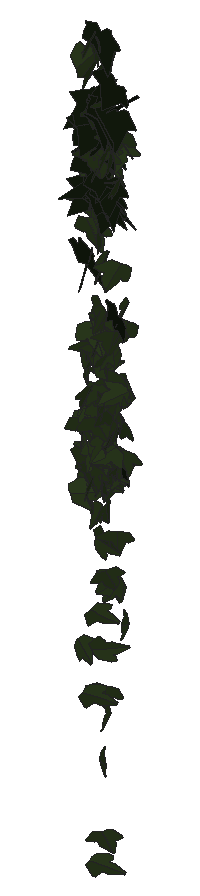
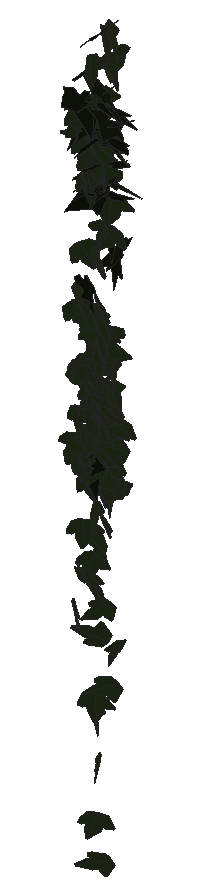
# SketchUp Ruby script. Lengths in inches.
U = 1.inch
M = Sketchup.active_model
def pt(a) = Geom::Point3d.new(a.map { |v| v * U })
def face(e, loops, mat)
  f = e.add_face(loops[0].map { |a| pt(a) })
  loops[1..].each { |l| e.add_face(l.map { |a| pt(a) }).erase! }
  f.material = f.back_material = mat if mat
  f
end
# faces: each face lists its corners as indices into pts; further lists are holes
def faces(e, pts, list, mat = nil) = list.each { |f| face(e, (f[0].is_a?(Array) ? f : [f]).map { |l| l.map { |i| pts[i] } }, mat) }
# xy, xz, yz: faces in a plane at the given z, y or x. An outline is a flat list of corners, or four numbers for a rectangle; further outlines are holes
def ring(l) = l.size == 4 ? [[l[0], l[1]], [l[2], l[1]], [l[2], l[3]], [l[0], l[3]]] : l.each_slice(2).to_a
def flat(e, list, mat, &to3) = list.each { |f| face(e, (f[0].is_a?(Array) ? f : [f]).map { |l| ring(l).map { |u, v| to3.(u, v) } }, mat) }
def xy(e, z, list, mat = nil) = flat(e, list, mat) { |x, y| [x, y, z] }
def xz(e, y, list, mat = nil) = flat(e, list, mat) { |x, z| [x, y, z] }
def yz(e, x, list, mat = nil) = flat(e, list, mat) { |y, z| [x, y, z] }
def lines(e, pts, list) = list.each { |a, b| e.add_line(pt(pts[a]), pt(pts[b])) }
# prism: a flat outline (further loops are holes) pulled along v
def prism(e, loops, v, mat = nil)
  f = face(e, loops, mat); d = Geom::Vector3d.new(v.map { |x| x * U })
  f.pushpull(f.normal.samedirection?(d) ? d.length : -d.length)
end
def box(e, o, s, mat = nil) = prism(e, [[o, [o[0] + s[0], o[1], o[2]], [o[0] + s[0], o[1] + s[1], o[2]], [o[0], o[1] + s[1], o[2]]]], [0, 0, s[2]], mat)
def at(x, y, z, deg = 0) = Geom::Transformation.translation(pt([x, y, z])) * Geom::Transformation.rotation(ORIGIN, Z_AXIS, deg.degrees)
def axes(o, x, y, z) = Geom::Transformation.new([*x, 0, *y, 0, *z, 0, *pt(o).to_a, 1])
def part(name) = M.definitions.add(name)
# library, detail: a bought-in or finely detailed component or shape, given as its bounding box
def library(name, o, s) = part(name).tap { |d| box(d.entities, o, s) }
def detail(e, o, s) = box(e.add_group.entities, o, s)
def put(e, d, t, mat = nil) = e.add_instance(d, t).tap { |i| i.material = mat if mat }
def group(e, t, mat = nil) = e.add_group.tap { |g| g.transformation = t; g.material = mat if mat }.entities
root = M.entities
M.materials.add("1026 AP 7946 SUNNY SIDE UP").color = [254, 231, 186]
M.materials.add("efeu1").color = [18, 25, 13]
M.materials.add("efeu2").color = [43, 57, 29]
c1 = part("ivyleaf_10")
p = [[0,0.5,-0.03],[-0.0625,2.02,-0.43],[-0.19,2.01,-0.46],[-0.54,1.05,-0.29],[-0.52,0.625,-0.18],[-0.83,0.76,-0.28],
  [-1.16,0.64,-0.33],[-1.15,0.33,-0.24],[-0.77,-0.39,0.02],[-0.3,-0.51,0.16],[0.04,-0.48,0.23],[-0.02,2.01,-0.4375],
  [-0.06,2.01,-0.43],[0.04,-0.49,0.23],[0.67,-0.49,0.14],[1.38,0.36,-0.2],[1.375,0.51,-0.24],[0.81,0.65,-0.19],
  [0.62,0.59,-0.15],[0.6,1.09,-0.28],[0.5,1.23,-0.31]]
faces(c1.entities,p,[[0,1,2,3,4,5,6,7,8,9,10],[11,12,0,13,14,15,16,17,18,19,20]],"efeu2")
c2 = part("ivyleaf_9")
p = [[1.54,2.16,1.25],[1.36,2.04,1.19],[-0.21,0.99,0.68],[-0.71,1.11,0.82],[-0.85,0.86,0.67],[-0.8,0.17,0.21],
  [-0.9,-0.01,0.1],[-0.67,-0.16,-0.02],[-0.08,-0.08,-0.05],[-0.03,-0.6,-0.4],[0.65,-0.88,-0.66],[0.83,-0.6,-0.49],
  [1.29,-0.42,-0.43],[1.8125,-0.07,-0.26],[1.21,0.44,0.15]]
faces(c2.entities,p,[[0,1,2,3,4,5,6,7,8,9,10,11,12,13,14]],"efeu1")
put(root,c1,axes([105.44,212.83,261.08],[-0.22128,-0.17573,0.01533],[0.00706,-0.02387,-0.2313],[0.27735,-0.1396,0.01812]),"1026 AP 7946 SUNNY SIDE UP")
put(root,c1,axes([105.27,212.93,260.67],[0.07124,-0.10081,0.19446],[0.19545,-0.14537,-0.11123],[0.27488,0.12949,0.0287]),"1026 AP 7946 SUNNY SIDE UP")
put(root,c1,axes([105.36,212.74,259.4],[-0.02708,0.1432,-0.1626],[-0.00095,-0.1592,-0.1489],[-0.33605,-0.01109,0.01352]),"1026 AP 7946 SUNNY SIDE UP")
put(root,c1,axes([105.4375,212.62,260.73],[0.03044,-0.01682,-0.23325],[-0.00065,0.22714,-0.0161],[0.35685,0.00185,0.01987]),"1026 AP 7946 SUNNY SIDE UP")
put(root,c1,axes([105.38,212.6,254.75],[0.00854,0.19841,0.07647],[-0.00793,0.07323,-0.20393],[-0.33238,0.00335,0.00683]),"1026 AP 7946 SUNNY SIDE UP")
put(root,c2,axes([105.5,212.76,266],[0.09763,0.17061,0.17604],[-0.03799,0.179,-0.17502],[-0.37671,0.02617,0.06327]),"1026 AP 7946 SUNNY SIDE UP")
put(root,c1,axes([105.26,212.79,258.43],[-0.15952,0.09823,-0.20296],[0.19847,-0.15252,-0.14578],[-0.28456,-0.16144,0.0121]),"1026 AP 7946 SUNNY SIDE UP")
put(root,c1,axes([105.46,212.78,264.3],[-0.30335,-0.14355,-0.00701],[0.02705,-0.01312,-0.24688],[0.22429,-0.19257,0.02029]),"1026 AP 7946 SUNNY SIDE UP")
put(root,c1,axes([105.53,212.83,258.88],[-0.20843,-0.10504,0.13226],[-0.05293,-0.14457,-0.15778],[0.25615,-0.11535,0.07502]),"1026 AP 7946 SUNNY SIDE UP")
put(root,c1,axes([105.48,212.68,260.21],[0.01512,-0.21436,0.03388],[0.00431,-0.03402,-0.22125],[0.34127,0.00993,0.00129]),"1026 AP 7946 SUNNY SIDE UP")
put(root,c1,axes([105.39,212.64,259.49],[-0.30371,-0.07569,-0.09097],[0.14534,0.00264,-0.21163],[0.11014,-0.21218,0.02842]),"1026 AP 7946 SUNNY SIDE UP")
put(root,c2,axes([105.56,212.89,264.43],[-0.3257,-0.11911,0.03771],[-0.02627,-0.04513,-0.24442],[0.19449,-0.20557,0.03014]),"1026 AP 7946 SUNNY SIDE UP")
put(root,c1,axes([105.47,212.86,261.24],[-0.33841,0.04416,-0.01506],[0.01648,-0.02262,-0.22553],[-0.07139,-0.21454,0.01935]),"1026 AP 7946 SUNNY SIDE UP")
put(root,c1,axes([105.55,212.65,257.8],[0.00414,0.04895,-0.20902],[-0.08657,0.19617,0.0491],[0.317,0.05293,0.01614]),"1026 AP 7946 SUNNY SIDE UP")
put(root,c2,axes([105.64,212.4,262.97],[-0.0648,0.0313,-0.2871],[-0.3536,0.16492,0.05427],[0.26394,0.22862,0.00222]),"1026 AP 7946 SUNNY SIDE UP")
put(root,c1,axes([105.51,212.99,258.33],[0.25702,0.11622,0.03653],[-0.07124,0.00431,0.20442],[0.17696,-0.16706,0.02924]),"1026 AP 7946 SUNNY SIDE UP")
put(root,c2,axes([105.625,212.85,266.29],[-0.38246,-0.04765,0.01537],[-0.01648,-0.02519,-0.25441],[0.0769,-0.2424,0.02193]),"1026 AP 7946 SUNNY SIDE UP")
put(root,c2,axes([105.28,212.68,263.21],[0.23413,-0.2247,-0.02069],[-0.02429,0.01232,-0.27755],[0.35372,0.14958,-0.00537]),"1026 AP 7946 SUNNY SIDE UP")
put(root,c1,axes([105.34,212.82,259.53],[0.32917,-0.00311,0.08997],[0.13655,-0.01825,-0.21519],[0.01555,0.2261,-0.0148]),"1026 AP 7946 SUNNY SIDE UP")
put(root,c1,axes([105.41,212.52,267.25],[0.06637,0.06134,-0.28287],[0.15017,0.25842,0.07602],[0.41669,-0.1029,0.01766]),"1026 AP 7946 SUNNY SIDE UP")
put(root,c1,axes([105.55,212.86,261.93],[0.16171,-0.18218,-0.10114],[-0.06315,0.0888,-0.21485],[0.31844,0.11013,0.00875]),"1026 AP 7946 SUNNY SIDE UP")
put(root,c1,axes([105.43,212.82,263.68],[-0.35081,0.02377,-0.08698],[0.11461,-0.07874,-0.22136],[-0.0771,-0.22522,0.06672]),"1026 AP 7946 SUNNY SIDE UP")
put(root,c1,axes([105.54,212.73,267.17],[0.10726,-0.24656,0.04116],[0.00872,-0.04137,-0.26373],[0.39302,0.06821,-0.00538]),"1026 AP 7946 SUNNY SIDE UP")
put(root,c1,axes([105.57,212.64,267.8125],[0.11867,-0.25043,-0.01937],[-0.01412,0.01544,-0.26933],[0.39448,0.07589,-0.00382]),"1026 AP 7946 SUNNY SIDE UP")
put(root,c2,axes([105.51,212.83,265.83],[-0.1649,-0.21075,0.08769],[-0.02069,-0.08926,-0.24151],[0.35749,-0.10237,0.02647]),"1026 AP 7946 SUNNY SIDE UP")
put(root,c1,axes([105.53,212.91,257.57],[0.22071,-0.14882,0.00739],[-0.00058,-0.01136,-0.21065],[0.23435,0.14013,-0.00748]),"1026 AP 7946 SUNNY SIDE UP")
put(root,c1,axes([105.55,212.68,258.3],[0.13075,-0.18767,0.04393],[0.02963,-0.03946,-0.2117],[0.30154,0.08526,0.00175]),"1026 AP 7946 SUNNY SIDE UP")
put(root,c2,axes([105.37,212.94,264.71],[0.17879,-0.21134,0.0306],[0.00684,-0.03271,-0.24713],[0.33577,0.1132,-0.01126]),"1026 AP 7946 SUNNY SIDE UP")
put(root,c1,axes([105.59,212.82,265.04],[0.1143,-0.21643,-0.10668],[-0.01175,0.10484,-0.23328],[0.37624,0.06902,0.02513]),"1026 AP 7946 SUNNY SIDE UP")
put(root,c1,axes([105.59,212.91,261.2],[0.09608,-0.21652,0.00671],[0.00368,-0.00738,-0.23181],[0.34065,0.06115,0.00061]),"1026 AP 7946 SUNNY SIDE UP")
put(root,c1,axes([105.625,213.03,253.6875],[-0.29514,-0.07377,0.01932],[-0.01723,-0.0243,-0.20703],[0.11861,-0.18711,0.01799]),"1026 AP 7946 SUNNY SIDE UP")
put(root,c1,axes([105.625,212.84,259.79],[0.10771,-0.20456,-0.06023],[-0.03818,0.05227,-0.22184],[0.33184,0.07241,-0.00597]),"1026 AP 7946 SUNNY SIDE UP")
put(root,c2,axes([105.79,212.77,266.65],[-0.18898,0.21599,0.03996],[-0.04326,0.02763,-0.25425],[-0.342,-0.12285,0.01008]),"1026 AP 7946 SUNNY SIDE UP")
put(root,c1,axes([105.6,212.85,259.82],[0.30425,-0.08417,-0.03252],[-0.05238,0.00122,-0.21702],[0.13101,0.19597,-0.01126]),"1026 AP 7946 SUNNY SIDE UP")
put(root,c2,axes([105.81,212.68,264.7],[-0.35867,0.08132,-0.01111],[-0.03158,-0.08747,-0.23251],[-0.12516,-0.21096,0.0905]),"1026 AP 7946 SUNNY SIDE UP")
put(root,c1,axes([105.54,212.78,259.67],[0.21054,0.16646,-0.02597],[-0.01059,-0.02809,-0.21988],[-0.26474,0.1335,-0.01185]),"1026 AP 7946 SUNNY SIDE UP")
put(root,c1,axes([105.38,212.49,258.05],[0.09678,-0.02241,-0.2198],[0.29038,0.11825,0.0428],[0.17129,-0.18781,0.05163]),"1026 AP 7946 SUNNY SIDE UP")
put(root,c1,axes([105.54,212.96,261.38],[0.2227,-0.16798,0.02163],[0.06951,0.00903,-0.22263],[0.25715,0.14304,0.04145]),"1026 AP 7946 SUNNY SIDE UP")
put(root,c2,axes([105.49,212.85,265.07],[-0.07743,-0.23381,-0.06941],[0.06074,0.059,-0.24448],[0.37717,-0.0575,0.02512]),"1026 AP 7946 SUNNY SIDE UP")
put(root,c2,axes([105.8,212.6875,265.68],[-0.25575,0.18251,-0.01538],[-0.0019,-0.02242,-0.25146],[-0.28807,-0.16189,0.01531]),"1026 AP 7946 SUNNY SIDE UP")
put(root,c1,axes([105.69,212.92,259.87],[0.08485,-0.16349,-0.13708],[-0.07215,0.12397,-0.1766],[0.32256,0.07074,-0.00344]),"1026 AP 7946 SUNNY SIDE UP")
put(root,c1,axes([105.62,212.57,258.61],[-0.32865,0.03345,-0.02605],[0.03395,-0.02551,-0.21707],[-0.05674,-0.20901,0.02105]),"1026 AP 7946 SUNNY SIDE UP")
put(root,c1,axes([105.35,212.79,258.18],[0.03251,0.02249,0.24878],[0.30742,0.14166,-0.03002],[-0.22534,0.19651,-0.00507]),"1026 AP 7946 SUNNY SIDE UP")
put(root,c1,axes([105.65,212.72,261.35],[0.13984,-0.21069,-0.07232],[-0.01219,0.07134,-0.2343],[0.34839,0.08706,0.02083]),"1026 AP 7946 SUNNY SIDE UP")
put(root,c1,axes([105.79,212.84,261.62],[-0.30331,0.05361,0.11483],[-0.19069,-0.04409,-0.19515],[-0.03598,-0.21822,0.06623]),"1026 AP 7946 SUNNY SIDE UP")
put(root,c1,axes([105.68,212.84,261.125],[-0.18243,-0.18461,0.0588],[-0.00916,-0.06441,-0.22309],[0.30419,-0.11266,0.02855]),"1026 AP 7946 SUNNY SIDE UP")
put(root,c1,axes([105.47,212.87,264.99],[0.28176,0.13939,0.10132],[0.13664,0.04683,-0.23308],[-0.22999,0.19858,-0.01435]),"1026 AP 7946 SUNNY SIDE UP")
put(root,c1,axes([105.71,212.8,252.27],[-0.09485,0.12016,0.15773],[-0.1359,0.12629,-0.13706],[-0.27326,-0.10451,0.01341]),"1026 AP 7946 SUNNY SIDE UP")
put(root,c1,axes([105.61,212.85,258.3],[-0.13688,0.17784,-0.05397],[0.01805,-0.05371,-0.20386],[-0.2914,-0.08686,0.01273]),"1026 AP 7946 SUNNY SIDE UP")
put(root,c1,axes([105.67,212.84,258.21],[0.10369,-0.20167,-0.01],[-0.00579,0.00781,-0.21854],[0.31734,0.06604,-0.00072]),"1026 AP 7946 SUNNY SIDE UP")
put(root,c1,axes([105.7,212.62,267.71],[0.23168,-0.17596,-0.13413],[-0.04584,0.13861,-0.22793],[0.34018,0.13852,0.06063]),"1026 AP 7946 SUNNY SIDE UP")
put(root,c2,axes([105.46,212.87,265.7],[-0.13789,-0.1389,-0.19304],[0.28735,0.08225,-0.15107],[0.22632,-0.18906,0.07419]),"1026 AP 7946 SUNNY SIDE UP")
put(root,c1,axes([105.7,212.84,261.43],[-0.28965,-0.12276,-0.00066],[0.01501,-0.01443,-0.22744],[0.19245,-0.18365,0.01675]),"1026 AP 7946 SUNNY SIDE UP")
put(root,c1,axes([105.65,212.69,259],[0.16619,0.16723,-0.09234],[-0.05843,-0.08348,-0.20392],[-0.29329,0.11139,-0.0117]),"1026 AP 7946 SUNNY SIDE UP")
put(root,c1,axes([105.68,212.92,259.67],[-0.28669,-0.11341,-0.01529],[0.04923,-0.02385,-0.21808],[0.17284,-0.18131,0.03676]),"1026 AP 7946 SUNNY SIDE UP")
put(root,c1,axes([105.7,212.77,259.82],[0.16729,0.16243,-0.09678],[-0.10342,-0.06998,-0.19985],[-0.2771,0.12418,0.01616]),"1026 AP 7946 SUNNY SIDE UP")
put(root,c1,axes([105.64,212.81,259.72],[0.36752,0.02151,-0.00868],[-0.01043,-0.02089,-0.24103],[-0.03487,0.23295,-0.01942]),"1026 AP 7946 SUNNY SIDE UP")
put(root,c1,axes([105.47,212.55,258.98],[-0.19521,-0.02606,-0.19883],[0.3051,0.00098,-0.1288],[0.02348,-0.22935,0.02068]),"1026 AP 7946 SUNNY SIDE UP")
put(root,c1,axes([105.54,212.73,261.52],[0.29677,0.12947,0.07025],[0.10553,0.02096,-0.23477],[-0.20385,0.19933,-0.01927]),"1026 AP 7946 SUNNY SIDE UP")
put(root,c1,axes([105.88,212.7,260.24],[-0.26732,-0.01176,0.14184],[-0.20106,-0.06964,-0.16911],[0.08266,-0.20743,0.04738]),"1026 AP 7946 SUNNY SIDE UP")
put(root,c1,axes([105.66,212.77,259.4],[0.04673,-0.20678,-0.04953],[0.0857,0.05322,-0.20583],[0.3222,0.01584,0.06193]),"1026 AP 7946 SUNNY SIDE UP")
put(root,c1,axes([105.76,212.91,265.17],[-0.22954,-0.18934,0.05011],[-0.00328,-0.06051,-0.24407],[0.30779,-0.14185,0.03477]),"1026 AP 7946 SUNNY SIDE UP")
put(root,c1,axes([105.68,212.68,263.65],[0.17551,-0.17899,-0.13159],[0.0416,0.15213,-0.19649],[0.34231,0.07328,0.09134]),"1026 AP 7946 SUNNY SIDE UP")
put(root,c1,axes([105.72,213,267.26],[0.01297,-0.24213,-0.06823],[0.03226,0.06532,-0.24818],[0.39282,0.00263,0.02263]),"1026 AP 7946 SUNNY SIDE UP")
put(root,c1,axes([105.71,212.9,257.6875],[0.03121,-0.19628,-0.06063],[0.05312,0.06036,-0.19906],[0.31729,0.0092,0.03929]),"1026 AP 7946 SUNNY SIDE UP")
put(root,c1,axes([105.76,212.67,266.39],[-0.07212,-0.25224,0.00935],[0.00499,-0.01125,-0.26413],[0.39694,-0.04569,0.00502]),"1026 AP 7946 SUNNY SIDE UP")
put(root,c1,axes([105.68,212.9,263.01],[0.18163,-0.17997,0.11615],[0.07411,-0.10461,-0.22038],[0.32648,0.12386,-0.01459]),"1026 AP 7946 SUNNY SIDE UP")
put(root,c1,axes([105.73,212.71,264.68],[0.20142,-0.2197,0.05315],[0.0154,-0.05529,-0.26159],[0.35498,0.12706,-0.01881]),"1026 AP 7946 SUNNY SIDE UP")
put(root,c2,axes([105.58,213.02,265.67],[0.10509,-0.21914,-0.08396],[-0.02049,0.07985,-0.23532],[0.36639,0.06732,0.01092]),"1026 AP 7946 SUNNY SIDE UP")
put(root,c1,axes([105.78,212.6,265.4],[-0.35455,-0.1182,-0.01023],[0.02885,-0.01514,-0.26139],[0.18419,-0.22517,0.02125]),"1026 AP 7946 SUNNY SIDE UP")
put(root,c2,axes([105.86,212.92,258.6875],[0.22062,0.00839,-0.2021],[-0.30364,-0.03807,-0.14415],[-0.0563,0.2382,-0.01449]),"1026 AP 7946 SUNNY SIDE UP")
put(root,c1,axes([105.6,212.56,253.79],[-0.11231,-0.06712,-0.1954],[0.25288,0.10123,-0.0989],[0.18916,-0.17518,0.0162]),"1026 AP 7946 SUNNY SIDE UP")
put(root,c1,axes([105.83,212.81,253.3],[0.09239,-0.18145,-0.09849],[-0.05036,0.08902,-0.19595],[0.31778,0.06686,-0.00242]),"1026 AP 7946 SUNNY SIDE UP")
put(root,c1,axes([105.84,212.67,258.41],[-0.15414,0.16749,0.06277],[-0.11099,0.02624,-0.19419],[-0.25677,-0.11189,0.04626]),"1026 AP 7946 SUNNY SIDE UP")
put(root,c1,axes([105.67,212.67,255.52],[-0.1223,-0.10744,-0.17196],[0.19701,0.11165,-0.13402],[0.24107,-0.14575,0.02228]),"1026 AP 7946 SUNNY SIDE UP")
put(root,c2,axes([105.66,212.84,267.83],[0.01478,-0.25847,0.0371],[-0.00259,-0.03757,-0.26665],[0.41066,0.00907,-0.00302]),"1026 AP 7946 SUNNY SIDE UP")
put(root,c1,axes([105.82,212.66,261.93],[0.20302,-0.18658,-0.03932],[-0.03314,0.03055,-0.23357],[0.29728,0.13082,0.00082]),"1026 AP 7946 SUNNY SIDE UP")
put(root,c1,axes([105.88,212.83,258.56],[-0.14367,0.1788,0.05168],[-0.14008,0.00572,-0.19205],[-0.25573,-0.10359,0.07617]),"1026 AP 7946 SUNNY SIDE UP")
put(root,c1,axes([105.78,212.75,261.13],[0.31645,-0.10306,0.01238],[0.00359,-0.02309,-0.2322],[0.16322,0.20032,-0.01889]),"1026 AP 7946 SUNNY SIDE UP")
put(root,c1,axes([105.55,212.92,256.89],[-0.05227,0.02222,0.24345],[0.35872,-0.06242,0.03876],[0.10231,0.23021,-0.01153]),"1026 AP 7946 SUNNY SIDE UP")
put(root,c1,axes([105.63,212.74,250.11],[-0.10531,-0.05523,-0.18963],[0.27345,0.06477,-0.08497],[0.12749,-0.18455,0.02562]),"1026 AP 7946 SUNNY SIDE UP")
put(root,c2,axes([105.6875,212.76,266.13],[0.03173,-0.23224,0.09141],[-0.00011,-0.09035,-0.24056],[0.39166,0.01879,-0.00747]),"1026 AP 7946 SUNNY SIDE UP")
put(root,c1,axes([105.87,212.55,260.13],[0.18328,-0.15919,-0.10779],[-0.04038,0.10738,-0.19886],[0.29602,0.11321,0.03962]),"1026 AP 7946 SUNNY SIDE UP")
put(root,c1,axes([105.88,212.92,258.26],[-0.14719,-0.1728,0.05221],[-0.00739,-0.05585,-0.20154],[0.28349,-0.09117,0.02186]),"1026 AP 7946 SUNNY SIDE UP")
put(root,c1,axes([105.71,212.78,258.86],[0.18207,-0.10262,0.16717],[0.17426,-0.11984,-0.15968],[0.24746,0.15989,-0.01055]),"1026 AP 7946 SUNNY SIDE UP")
put(root,c1,axes([105.96,212.87,256.18],[0.28464,-0.1046,-0.12753],[-0.17573,0.0526,-0.21488],[0.18357,0.21255,-0.00796]),"1026 AP 7946 SUNNY SIDE UP")
put(root,c1,axes([105.875,212.7,259.2],[0.14901,0.13785,-0.14507],[-0.11519,-0.12134,-0.17292],[-0.2886,0.11961,-0.00589]),"1026 AP 7946 SUNNY SIDE UP")
put(root,c1,axes([105.8,212.55,259.7],[-0.25755,-0.16208,-0.09159],[0.12527,0.04394,-0.23593],[0.26153,-0.18066,0.02282]),"1026 AP 7946 SUNNY SIDE UP")
put(root,c1,axes([105.86,212.96,258.51],[-0.07485,-0.11851,0.16217],[0.0293,-0.16458,-0.12228],[0.30929,-0.01309,0.05083]),"1026 AP 7946 SUNNY SIDE UP")
put(root,c1,axes([105.93,212.91,260.09],[0.12838,-0.16306,-0.12463],[-0.08839,0.10611,-0.18723],[0.30588,0.0991,-0.00179]),"1026 AP 7946 SUNNY SIDE UP")
put(root,c1,axes([105.9,212.84,264.65],[-0.15409,-0.22399,0.00098],[0.01203,-0.00577,-0.25172],[0.35201,-0.09785,0.00903]),"1026 AP 7946 SUNNY SIDE UP")
put(root,c1,axes([105.8125,212.65,260.82],[0.03532,-0.00074,0.23556],[0.00505,0.22974,0.00179],[-0.35952,0.00316,0.02316]),"1026 AP 7946 SUNNY SIDE UP")
put(root,c1,axes([105.89,212.93,259.28],[-0.00796,-0.20859,-0.04954],[0.01367,0.04668,-0.21454],[0.33589,-0.00684,0.00756]),"1026 AP 7946 SUNNY SIDE UP")
put(root,c1,axes([105.64,212.9375,258.56],[0.17513,0.0272,0.17597],[0.26014,0.04189,-0.11786],[-0.07853,0.19944,0.002]),"1026 AP 7946 SUNNY SIDE UP")
put(root,c1,axes([105.93,212.73,260.68],[-0.34339,-0.00294,0.02329],[-0.0349,-0.023,-0.22393],[0.00829,-0.21835,0.02198]),"1026 AP 7946 SUNNY SIDE UP")
put(root,c1,axes([105.87,212.87,260.19],[-0.08582,-0.20689,-0.03054],[0.05828,0.01936,-0.21805],[0.32317,-0.05844,0.03121]),"1026 AP 7946 SUNNY SIDE UP")
put(root,c1,axes([105.89,212.76,265.46],[0.11715,-0.22431,0.07234],[0.01978,-0.07109,-0.24369],[0.36966,0.07489,-0.00989]),"1026 AP 7946 SUNNY SIDE UP")
put(root,c1,axes([105.89,212.92,261.78],[-0.2745,0.13573,-0.02631],[0.00647,-0.03726,-0.22636],[-0.2173,-0.17257,0.02649]),"1026 AP 7946 SUNNY SIDE UP")
put(root,c1,axes([105.65,212.87,265.32],[0.28008,0.01213,0.1789],[0.27191,0.01535,-0.18382],[-0.0305,0.24824,0.00409]),"1026 AP 7946 SUNNY SIDE UP")
put(root,c2,axes([105.7,212.85,264.4],[0.36284,-0.07611,-0.0014],[-0.01432,-0.02466,-0.249],[0.11883,0.22944,-0.02573]),"1026 AP 7946 SUNNY SIDE UP")
put(root,c1,axes([105.94,212.88,260.52],[-0.14462,-0.20128,0.02611],[0.00688,-0.03104,-0.22751],[0.31915,-0.09054,0.01673]),"1026 AP 7946 SUNNY SIDE UP")
put(root,c2,axes([106.03,212.95,266.38],[-0.02246,0.24952,-0.01696],[-0.00298,-0.01802,-0.25756],[-0.39334,-0.01411,0.00292]),"1026 AP 7946 SUNNY SIDE UP")
put(root,c1,axes([106.01,212.66,259.11],[0.29327,-0.01055,-0.11936],[-0.18281,-0.01234,-0.19181],[0.00383,0.21919,-0.01525]),"1026 AP 7946 SUNNY SIDE UP")
put(root,c1,axes([105.93,213,258.64],[0.16954,-0.17442,-0.00351],[-0.00202,0.00205,-0.21123],[0.27427,0.10783,0.00062]),"1026 AP 7946 SUNNY SIDE UP")
put(root,c2,axes([105.88,212.78,264.38],[-0.11526,-0.22783,0.04637],[-0.01929,-0.04469,-0.24681],[0.36505,-0.07429,0.0016]),"1026 AP 7946 SUNNY SIDE UP")
put(root,c1,axes([105.9,212.95,258.52],[0.31181,-0.04079,0.0034],[-0.00037,-0.01859,-0.20783],[0.06437,0.19746,-0.01765]),"1026 AP 7946 SUNNY SIDE UP")
put(root,c2,axes([105.8,212.75,266.34],[0.02956,-0.25303,0.03258],[0.0012,-0.03309,-0.26158],[0.40125,0.01874,-0.00162]),"1026 AP 7946 SUNNY SIDE UP")
put(root,c1,axes([105.92,212.6,250.86],[-0.23222,-0.12732,-0.06276],[0.0878,0.02714,-0.20011],[0.2033,-0.15716,0.01474]),"1026 AP 7946 SUNNY SIDE UP")
put(root,c1,axes([106,212.86,265.72],[-0.27678,-0.17845,0.01127],[0.00776,-0.02161,-0.25763],[0.28111,-0.1751,0.0182]),"1026 AP 7946 SUNNY SIDE UP")
put(root,c2,axes([105.8125,212.58,264.59],[0.16154,-0.18341,-0.14312],[-0.06961,0.13239,-0.21462],[0.35402,0.10972,0.02311]),"1026 AP 7946 SUNNY SIDE UP")
put(root,c1,axes([105.98,212.87,256.1875],[0.2916,-0.15347,-0.03363],[-0.05769,0.00534,-0.24717],[0.23959,0.18807,-0.01859]),"1026 AP 7946 SUNNY SIDE UP")
put(root,c2,axes([105.88,212.76,264.79],[-0.08879,-0.23598,-0.00086],[0.00408,-0.00114,-0.24996],[0.37104,-0.05646,0.00254]),"1026 AP 7946 SUNNY SIDE UP")
put(root,c1,axes([106.22,212.8,260.4375],[-0.10906,0.01754,0.21638],[-0.31338,-0.07711,-0.06165],[0.10737,-0.20722,0.03987]),"1026 AP 7946 SUNNY SIDE UP")
put(root,c1,axes([106.1,212.89,258.94],[-0.1874,-0.09533,0.14458],[-0.12859,-0.11873,-0.15473],[0.23455,-0.14127,0.03069]),"1026 AP 7946 SUNNY SIDE UP")
put(root,c1,axes([106.07,212.79,265.875],[-0.37423,-0.0425,0.06332],[-0.08944,-0.03128,-0.24838],[0.07668,-0.24387,0.01933]),"1026 AP 7946 SUNNY SIDE UP")
put(root,c2,axes([105.87,212.86,265.9375],[0.31699,-0.09895,-0.11559],[-0.16331,0.04163,-0.23098],[0.16838,0.22665,-0.00642]),"1026 AP 7946 SUNNY SIDE UP")
put(root,c1,axes([105.96,212.86,265.42],[-0.1596,-0.22301,-0.0115],[0.07609,-0.01137,-0.24745],[0.34266,-0.10135,0.04959]),"1026 AP 7946 SUNNY SIDE UP")
put(root,c1,axes([105.79,212.625,254.77],[-0.09789,-0.05119,0.1963],[0.20817,0.13772,0.08336],[-0.23063,0.14604,-0.00808]),"1026 AP 7946 SUNNY SIDE UP")
put(root,c1,axes([105.95,212.67,256.4375],[-0.18514,-0.16265,-0.08627],[0.09067,0.06036,-0.20622],[0.27229,-0.13069,0.01001]),"1026 AP 7946 SUNNY SIDE UP")
put(root,c1,axes([106.04,212.77,261.16],[0.22353,-0.16615,-0.05815],[-0.07706,0.03091,-0.22444],[0.26445,0.14945,-0.01624]),"1026 AP 7946 SUNNY SIDE UP")
put(root,c1,axes([106.04,212.86,257.2],[-0.23227,-0.14513,-0.00243],[0.01441,-0.00714,-0.21304],[0.22776,-0.14755,0.011]),"1026 AP 7946 SUNNY SIDE UP")
put(root,c1,axes([106.13,212.91,259.61],[-0.2455,0.1154,0.09717],[-0.14164,0.03459,-0.19838],[-0.1859,-0.17876,0.02283]),"1026 AP 7946 SUNNY SIDE UP")
put(root,c2,axes([105.91,212.76,264.57],[-0.00466,-0.24406,0.04609],[0.00285,-0.04615,-0.2517],[0.39054,-0.00258,0.00239]),"1026 AP 7946 SUNNY SIDE UP")
put(root,c1,axes([106.05,212.62,259.47],[0.11061,-0.19738,-0.02779],[-0.00968,0.02525,-0.2157],[0.31286,0.07056,0.00315]),"1026 AP 7946 SUNNY SIDE UP")
put(root,c1,axes([106.07,212.96,258.65],[-0.02532,-0.20613,-0.01178],[0.0019,0.0102,-0.21294],[0.32452,-0.01614,0.00033]),"1026 AP 7946 SUNNY SIDE UP")
put(root,c1,axes([105.95,212.86,265.5625],[0.35641,0.10456,0.01804],[0.03679,-0.01046,-0.25645],[-0.16244,0.22706,-0.01851]),"1026 AP 7946 SUNNY SIDE UP")
put(root,c1,axes([106.02,212.61,259.93],[-0.1206,-0.17026,-0.13724],[0.098,0.11686,-0.19155],[0.32451,-0.09856,0.00685]),"1026 AP 7946 SUNNY SIDE UP")
put(root,c1,axes([106.07,212.59,265.52],[0.11329,-0.17585,-0.16436],[0.00667,0.16666,-0.18747],[0.37225,0.05053,0.05338]),"1026 AP 7946 SUNNY SIDE UP")
put(root,c2,axes([106,212.8125,266.86],[-0.11116,-0.1834,0.16873],[-0.0171,-0.16899,-0.19949],[0.38735,-0.06009,0.03962]),"1026 AP 7946 SUNNY SIDE UP")
put(root,c1,axes([106.125,212.62,261.63],[-0.20415,-0.17971,0.02412],[-0.00645,-0.02713,-0.2282],[0.28511,-0.1293,0.01211]),"1026 AP 7946 SUNNY SIDE UP")
put(root,c1,axes([106.15,212.72,263.02],[-0.19497,-0.17474,0.11137],[-0.01166,-0.12347,-0.21313],[0.32371,-0.10969,0.0594]),"1026 AP 7946 SUNNY SIDE UP")
put(root,c1,axes([106.12,212.76,264.85],[0.08986,-0.23489,-0.04424],[-0.00091,0.04265,-0.24861],[0.37509,0.05638,0.01]),"1026 AP 7946 SUNNY SIDE UP")
put(root,c1,axes([106.06,212.9,260.32],[0.29874,-0.1012,0.0214],[0.01785,-0.02397,-0.22131],[0.16165,0.18968,-0.01511]),"1026 AP 7946 SUNNY SIDE UP")
put(root,c1,axes([106.02,212.79,260.24],[0.30368,-0.08158,0.06187],[0.08423,-0.02865,-0.21608],[0.13569,0.20035,-0.00432]),"1026 AP 7946 SUNNY SIDE UP")
put(root,c2,axes([106.04,212.8125,266.27],[-0.08336,-0.24249,0.01705],[0.00138,-0.01853,-0.25578],[0.38234,-0.05281,0.00464]),"1026 AP 7946 SUNNY SIDE UP")
put(root,c1,axes([106.26,212.75,260.38],[-0.15875,-0.05713,0.19455],[-0.11507,-0.18651,-0.09935],[0.28862,-0.10578,0.06739]),"1026 AP 7946 SUNNY SIDE UP")
put(root,c2,axes([106.28,212.53,262.14],[0.12936,-0.02003,-0.23313],[-0.35487,0.01929,-0.08621],[0.03934,0.23991,-0.01111]),"1026 AP 7946 SUNNY SIDE UP")
put(root,c1,axes([106.16,212.9,262.12],[0.13862,-0.2128,0.00472],[-0.00765,-0.00827,-0.23721],[0.33464,0.08796,-0.00737]),"1026 AP 7946 SUNNY SIDE UP")
put(root,c1,axes([106.18,212.72,261.74],[0.14905,-0.2078,-0.04331],[-0.04069,0.03307,-0.23489],[0.33051,0.09778,-0.00938]),"1026 AP 7946 SUNNY SIDE UP")
put(root,c1,axes([106.16,212.58,259.66],[0.18156,-0.18351,-0.04582],[-0.01317,0.04589,-0.2224],[0.29623,0.11451,0.0182]),"1026 AP 7946 SUNNY SIDE UP")
put(root,c1,axes([106.23,212.86,255.39],[0.07349,-0.13422,-0.16775],[-0.08597,0.15258,-0.14552],[0.31952,0.07192,-0.00057]),"1026 AP 7946 SUNNY SIDE UP")
put(root,c1,axes([106.19,212.96,258.78],[-0.08126,-0.19536,0.04795],[-0.00762,-0.04798,-0.20832],[0.3161,-0.05138,0.0073]),"1026 AP 7946 SUNNY SIDE UP")
put(root,c1,axes([106.16,212.85,258.98],[-0.32259,-0.02866,-0.02412],[0.04202,-0.02479,-0.21158],[0.04003,-0.20498,0.02773]),"1026 AP 7946 SUNNY SIDE UP")
put(root,c1,axes([106.24,212.82,261.78],[-0.19789,-0.1632,0.10119],[-0.03378,-0.10589,-0.20827],[0.29836,-0.12024,0.04354]),"1026 AP 7946 SUNNY SIDE UP")
